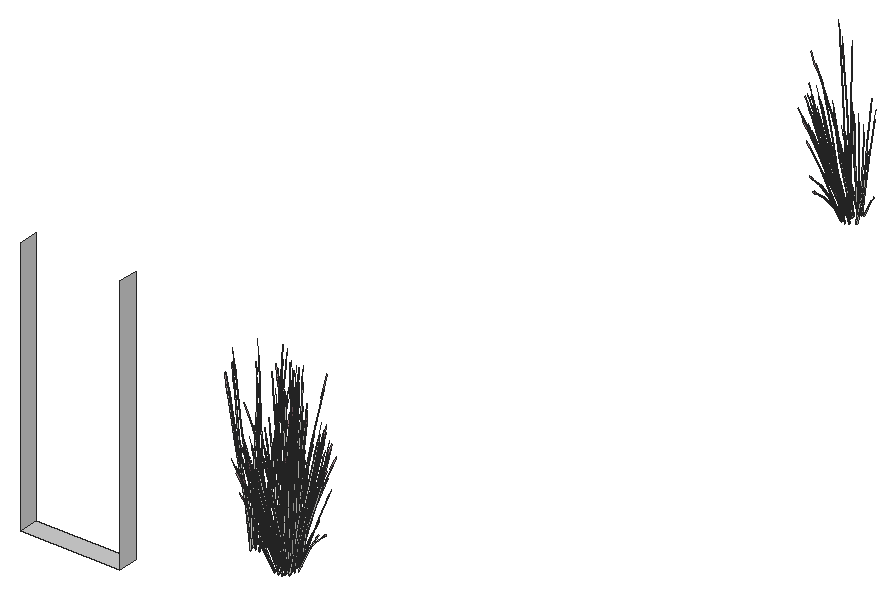
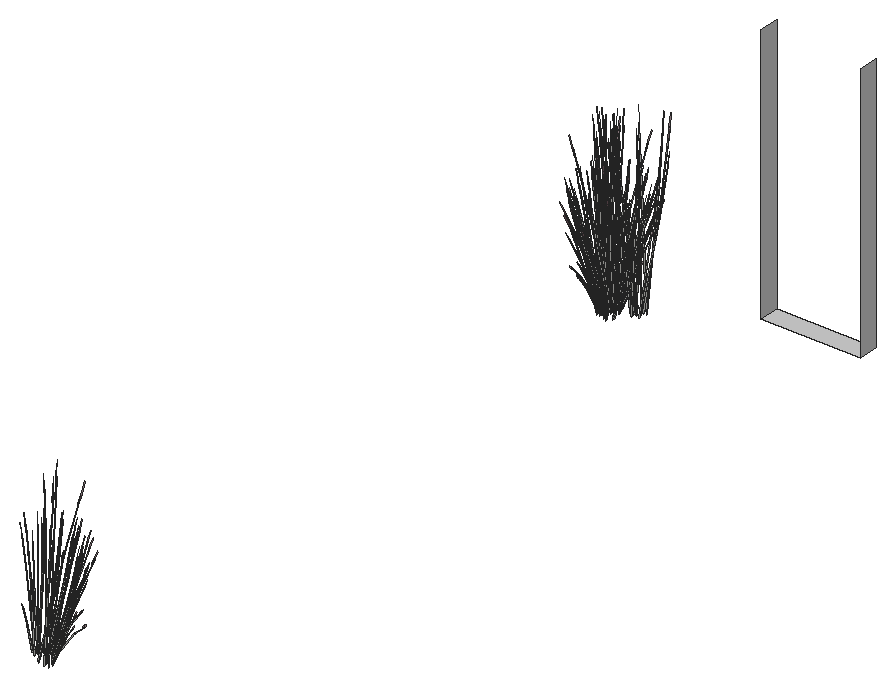
# SketchUp Ruby script. Lengths in inches.
U = 1.inch
M = Sketchup.active_model
def pt(a) = Geom::Point3d.new(a.map { |v| v * U })
def face(e, loops, mat)
  f = e.add_face(loops[0].map { |a| pt(a) })
  loops[1..].each { |l| e.add_face(l.map { |a| pt(a) }).erase! }
  f.material = f.back_material = mat if mat
  f
end
# faces: each face lists its corners as indices into pts; further lists are holes
def faces(e, pts, list, mat = nil) = list.each { |f| face(e, (f[0].is_a?(Array) ? f : [f]).map { |l| l.map { |i| pts[i] } }, mat) }
# xy, xz, yz: faces in a plane at the given z, y or x. An outline is a flat list of corners, or four numbers for a rectangle; further outlines are holes
def ring(l) = l.size == 4 ? [[l[0], l[1]], [l[2], l[1]], [l[2], l[3]], [l[0], l[3]]] : l.each_slice(2).to_a
def flat(e, list, mat, &to3) = list.each { |f| face(e, (f[0].is_a?(Array) ? f : [f]).map { |l| ring(l).map { |u, v| to3.(u, v) } }, mat) }
def xy(e, z, list, mat = nil) = flat(e, list, mat) { |x, y| [x, y, z] }
def xz(e, y, list, mat = nil) = flat(e, list, mat) { |x, z| [x, y, z] }
def yz(e, x, list, mat = nil) = flat(e, list, mat) { |y, z| [x, y, z] }
def lines(e, pts, list) = list.each { |a, b| e.add_line(pt(pts[a]), pt(pts[b])) }
# prism: a flat outline (further loops are holes) pulled along v
def prism(e, loops, v, mat = nil)
  f = face(e, loops, mat); d = Geom::Vector3d.new(v.map { |x| x * U })
  f.pushpull(f.normal.samedirection?(d) ? d.length : -d.length)
end
def box(e, o, s, mat = nil) = prism(e, [[o, [o[0] + s[0], o[1], o[2]], [o[0] + s[0], o[1] + s[1], o[2]], [o[0], o[1] + s[1], o[2]]]], [0, 0, s[2]], mat)
def at(x, y, z, deg = 0) = Geom::Transformation.translation(pt([x, y, z])) * Geom::Transformation.rotation(ORIGIN, Z_AXIS, deg.degrees)
def axes(o, x, y, z) = Geom::Transformation.new([*x, 0, *y, 0, *z, 0, *pt(o).to_a, 1])
def part(name) = M.definitions.add(name)
# library, detail: a bought-in or finely detailed component or shape, given as its bounding box
def library(name, o, s) = part(name).tap { |d| box(d.entities, o, s) }
def detail(e, o, s) = box(e.add_group.entities, o, s)
def put(e, d, t, mat = nil) = e.add_instance(d, t).tap { |i| i.material = mat if mat }
def group(e, t, mat = nil) = e.add_group.tap { |g| g.transformation = t; g.material = mat if mat }.entities
root = M.entities
M.materials.add("LightPink_Translucent").color = [144, 107, 117]
M.materials["LightPink_Translucent"].alpha = 0.75
M.materials.add("[Cladding_Siding_White]1").color = [207, 207, 207]
c1 = part("blade")
p = [[2.15,0.21,22],[0,0.17,0],[0.09,0.45,0],[2.18,0.31,22],[2.29,0.31,22],[0.38,0.45,0],
  [2.48,0.24,33],[2.49,0.24,33],[2.48,0.22,33]]
faces(c1.entities,p,[[0,1,2,3],[4,5,2,3],[6,3,4,7],[8,0,3,6]])
c2 = part("seeds")
p = [[0.3,-0.1,1.38],[-0.01,-0.03,1.59],[-0.01,-0.03,0.03],[0.14,-0.07,-0.07],[0.29,-0.03,3],[0.15,0.01,3.11]]
faces(c2.entities,p,[[0,1,2,3],[1,0,4,5]],"LightPink_Translucent")
c3 = part("blade with seeds")
put(c3.entities,c1,at(0,0,0))
put(c3.entities,c2,axes([2.4,0.25,30.99],[1.5799,-0.05474,1.17369],[-0.12525,1.92788,0.29478],[-0.07173,-0.02425,1.56792]))
xy(root,153,[[312,87,342,93]],"[Cladding_Siding_White]1")
yz(root,312,[[87,153,93,231]],"[Cladding_Siding_White]1")
yz(root,342,[[87,153,93,231]],"[Cladding_Siding_White]1")
put(root,c3,axes([371.09,110.03,153.64],[0.11194,0.19382,1.61094],[-0.51725,0.16318,0.13026],[-0.1169,-0.30428,0.68866]))
put(root,c3,axes([373.11,109.75,152.44],[-0.13919,0.12219,1.34422],[-0.41687,-0.21387,-0.28909],[0.07727,-0.26598,0.57472]))
put(root,c3,axes([372.47,110.17,154.68],[-0.23372,-0.49086,-0.66783],[0.48111,-0.27356,0.08059],[-0.05465,-0.23717,0.9447]))
put(root,c3,axes([370.95,109.51,152.44],[-0.02965,0.19748,1.34422],[-0.43351,0.16532,-0.28909],[-0.10133,-0.25525,0.57472]))
put(root,c3,axes([373.45,110.65,154.68],[0.01274,-0.55841,-0.66783],[0.53656,0.0375,0.08059],[0.05662,-0.23657,0.9447]))
put(root,c3,axes([372.52,109.75,154.25],[0.14763,-0.46424,-0.33289],[0.4307,0.1354,0.42977],[-0.03949,-0.18691,0.82232]))
put(root,c3,axes([372.84,110.37,153.64],[-0.09118,0.2075,1.61094],[-0.3825,-0.42941,0.13026],[0.17255,-0.26763,0.68866]))
put(root,c3,axes([372.3,110.07,154.4],[-0.48137,-0.15133,-0.48033],[0.165,-0.51886,-0.37205],[-0.04414,-0.2089,0.91906]))
put(root,c3,axes([372.59,108.77,152.6],[0.06282,0.35202,1.07969],[-0.34848,-0.19497,0.79328],[0.0375,-0.18025,0.23781]))
put(root,c3,axes([373.34,110.46,154.4],[-0.35055,-0.40562,-0.48033],[0.37031,-0.35523,-0.37205],[0.05334,-0.20609,0.91906]))
put(root,c3,axes([372.71,110.05,154.73],[-0.47919,0.28106,-0.11431],[-0.23549,-0.49884,-0.63445],[-0.06322,-0.21021,0.96403]))
put(root,c3,axes([373.7,110.68,154.73],[-0.53819,-0.02991,-0.11431],[0.01471,-0.56632,-0.63445],[0.03738,-0.21811,0.96403]))
put(root,c3,axes([373.67,110.31,154.25],[0.33133,-0.31784,-0.33289],[0.31365,0.36292,0.42977],[0.04772,-0.1844,0.82232]))
put(root,c3,axes([370.8,109.2,152.6],[0.25544,0.21011,1.07969],[-0.37201,0.1263,0.79328],[-0.0796,-0.16148,0.23781]))
put(root,c3,axes([371.42,110.31,154.68],[-0.41756,-0.29179,-0.66783],[0.29675,-0.51132,0.08059],[-0.15128,-0.17422,0.9447]))
put(root,c3,axes([371.28,109.92,154.25],[-0.07563,-0.48625,-0.33289],[0.43235,-0.1284,0.42977],[-0.11613,-0.13934,0.82232]))
put(root,c3,axes([362.35,112.01,155.67],[-0.2011,-0.61905,-0.65645],[0.5793,-0.22295,-0.17229],[-0.02223,-0.20963,1.449]))
put(root,c3,axes([370.34,110.63,153.64],[0.1819,0.10401,1.61094],[-0.37643,0.43634,0.13026],[-0.23461,-0.19684,0.68866]))
put(root,c3,axes([371.22,110.32,154.4],[-0.48321,0.1435,-0.48033],[-0.08453,-0.54345,-0.37205],[-0.12979,-0.15574,0.91906]))
put(root,c3,axes([374.08,111.62,154.68],[0.25579,-0.47633,-0.66783],[0.44823,0.33852,0.08059],[0.15273,-0.17258,0.9447]))
put(root,c3,axes([374.07,111.4,154.4],[-0.1258,-0.55122,-0.48033],[0.4764,-0.09643,-0.37205],[0.13652,-0.14806,0.91906]))
put(root,c3,axes([374.29,111.79,154.73],[-0.45297,-0.33287,-0.11431],[0.26096,-0.48206,-0.63445],[0.12798,-0.16757,0.96403]))
put(root,c3,axes([372.42,113.61,153.125],[0.42317,0.24343,1.42185],[-0.41456,0.52443,0.56227],[-0.18569,-0.31082,1.19198]))
put(root,c3,axes([361.17,111.93,155.59],[0,-0.60368,-0.46672],[0.54787,0,0],[0,-0.13749,1.48054]))
put(root,c3,axes([362.6875,110.14,155.59],[0.4583,-0.30184,-0.46672],[0.27394,0.54125,0],[0.10438,-0.06875,1.48054]))
put(root,c3,axes([374.45,111.18,152.44],[-0.17494,-0.01788,1.34422],[-0.17922,-0.47967,-0.28909],[0.21491,-0.13569,0.57472]))
put(root,c3,axes([363.23,111.38,155.63],[0.32983,-0.45375,-0.58612],[0.40974,0.41145,-0.15383],[0.13217,-0.11319,1.29375]))
put(root,c3,axes([374.65,110.3,152.6],[-0.16311,0.3073,1.07969],[-0.1402,-0.41288,0.79328],[0.13471,-0.10346,0.23781]))
put(root,c3,axes([374.42,111.46,154.25],[0.42626,-0.08628,-0.33289],[0.11256,0.4932,0.42977],[0.12215,-0.13247,0.82232]))
put(root,c3,axes([370.27,110.78,154.25],[-0.27863,-0.37797,-0.33289],[0.31815,-0.35779,0.42977],[-0.16164,-0.05444,0.82232]))
put(root,c3,axes([370.17,111.18,152.44],[0.09561,0.16807,1.34422],[-0.22031,0.45686,-0.28909],[-0.22622,-0.1092,0.57472]))
put(root,c3,axes([370.57,111.03,154.68],[-0.48951,-0.01454,-0.66783],[0.03288,-0.61207,0.08059],[-0.20738,-0.06459,0.9447]))
put(root,c3,axes([375.65,112.24,154.43],[0.06795,-0.09195,1.64448],[-0.08698,-0.56405,-0.26007],[0.1705,-0.10694,0.13189]))
put(root,c3,axes([370.41,111.15,154.4],[-0.35558,0.39989,-0.48033],[-0.31141,-0.42243,-0.37205],[-0.18066,-0.06084,0.91906]))
put(root,c3,axes([369.61,111.68,152.6],[0.31263,-0.0432,1.07969],[-0.19831,0.38061,0.79328],[-0.15449,-0.0571,0.23781]))
put(root,c3,axes([371.8125,112.04,152.56],[-0.53176,0.03727,0.42055],[-0.04809,-0.6186,-0.2024],[0.0952,-0.0627,1.35025]))
put(root,c3,axes([370.59,110.74,154.73],[-0.02622,0.61393,-0.11431],[-0.49645,-0.01678,-0.63445],[-0.1912,-0.04265,0.96403]))
put(root,c3,axes([370.44,112.49,152.33],[0,0.60368,0.46672],[-0.54787,0,0],[0,-0.13749,1.48054]))
put(root,c3,axes([374.31,113.09,154.73],[-0.24639,-0.54664,-0.11431],[0.43729,-0.26863,-0.63445],[0.18428,-0.07212,0.96403]))
put(root,c3,axes([374.29,112.62,154.4],[0.13266,-0.54912,-0.48033],[0.45484,0.18822,-0.37205],[0.18313,-0.05035,0.91906]))
put(root,c3,axes([369.96,111.58,153.64],[0.20312,-0.01367,1.61094],[-0.13474,0.59258,0.13026],[-0.28946,-0.03665,0.68866]))
put(root,c3,axes([371.6875,112.79,152.56],[-0.23759,0.54397,0.42055],[-0.49367,-0.26179,-0.2024],[0,-0.12539,1.35025]))
put(root,c3,axes([373.3,110.7,152.33],[-0.4583,-0.30184,0.46672],[0.27394,-0.54125,0],[0.10438,0.06875,1.48054]))
put(root,c3,axes([374.2,112.82,154.68],[0.4303,-0.26662,-0.66783],[0.23981,0.54882,0.08059],[0.20791,-0.06234,0.9447]))
put(root,c3,axes([362.43,113.17,155.63],[-0.50939,-0.09897,-0.58612],[0.10749,-0.61051,-0.15383],[-0.15202,-0.07398,1.29375]))
put(root,c3,axes([371.57,110.97,152.33],[-0.14146,0.59996,0.16584],[-0.51766,-0.16978,0.32981],[0.08942,-0.00292,1.50782]))
put(root,c3,axes([372.65,111.64,152.46],[0.09447,-0.53876,0.13611],[0.46155,0.09352,-0.38866],[0.084,0.05532,1.1914]))
put(root,c3,axes([372.45,111.78,152.56],[-0.29417,-0.5067,0.42055],[0.44558,-0.35681,-0.2024],[0.0952,0.0627,1.35025]))
put(root,c3,axes([371.52,114.07,152.33],[0.52621,-0.16023,0.16584],[0.12993,0.59629,0.32981],[-0.04693,-0.08688,1.50782]))
put(root,c3,axes([374.57,112.875,154.25],[0.40696,0.16841,-0.33289],[-0.1187,0.49132,0.42977],[0.16385,-0.04505,0.82232]))
put(root,c3,axes([361.76,114.32,155.59],[-0.4583,-0.30184,-0.46672],[0.27394,-0.54125,0],[-0.10438,-0.06875,1.48054]))
put(root,c3,axes([364.81,110.75,155.59],[0.4583,0.30184,-0.46672],[-0.27394,0.54125,0],[0.10438,0.06875,1.48054]))
put(root,c3,axes([369.78,112.09,154.25],[-0.40696,-0.16841,-0.33289],[0.1187,-0.49132,0.42977],[-0.16385,0.04505,0.82232]))
put(root,c3,axes([373.13,111.01,152.33],[-0.52621,0.16023,0.16584],[-0.12993,-0.59629,0.32981],[0.04693,0.08688,1.50782]))
put(root,c3,axes([373.46,112.26,153.64],[-0.20312,0.01367,1.61094],[0.13474,-0.59258,0.13026],[0.28946,0.03665,0.68866]))
put(root,c3,axes([372,113.43,152.46],[-0.09447,0.53876,0.13611],[-0.46155,-0.09352,-0.38866],[-0.084,-0.05532,1.1914]))
put(root,c3,axes([373.08,114.1,152.33],[0.14146,-0.59996,0.16584],[0.51766,0.16978,0.32981],[-0.08942,0.00292,1.50782]))
put(root,c3,axes([371.02,112.01,153.14],[0.13919,-0.08733,1.6644],[0.048,0.60974,0.13026],[-0.3015,0.08091,0.59487]))
put(root,c3,axes([373.89,112.57,152.33],[-0.38474,-0.43973,0.16584],[0.38772,-0.42651,0.32981],[-0.04249,0.0898,1.50782]))
put(root,c3,axes([364.14,111.91,155.63],[0.50939,0.09897,-0.58612],[-0.10749,0.61051,-0.15383],[0.15202,0.07398,1.29375]))
put(root,c3,axes([375.43,112.97,152.6],[-0.30256,0.09966,1.07969],[0.14242,-0.41189,0.79328],[0.16051,0.02818,0.23781]))
put(root,c3,axes([371.35,114.375,152.33],[0.4583,0.30184,0.46672],[-0.27394,0.54125,0],[-0.10438,-0.06875,1.48054]))
put(root,c3,axes([372.96,112.28,152.56],[0.23759,-0.54397,0.42055],[0.49367,0.26179,-0.2024],[0,0.12539,1.35025]))
put(root,c3,axes([369.53,112.42,154.43],[-0.07997,0.07838,1.64448],[0.0068,0.57266,-0.26007],[-0.1833,0.07447,0.13189]))
put(root,c3,axes([370.0625,112.34,154.4],[-0.13266,0.54912,-0.48033],[-0.45484,-0.18822,-0.37205],[-0.18313,0.05035,0.91906]))
put(root,c3,axes([370.04,111.87,154.73],[0.24639,0.54664,-0.11431],[-0.43729,0.26863,-0.63445],[-0.18428,0.07212,0.96403]))
put(root,c3,axes([374.9,114.24,153.69],[-0.09372,-0.50747,-0.03282],[0.44299,-0.11666,-0.14882],[0.09251,0.03217,0.49085]))
put(root,c3,axes([373.75,114.23,154.73],[0.02622,-0.61393,-0.11431],[0.49645,0.01678,-0.63445],[0.1912,0.04265,0.96403]))
put(root,c3,axes([374.21,112.59,152.33],[0,-0.60368,0.46672],[0.54787,0,0],[0,0.13749,1.48054]))
put(root,c3,axes([372.83,113.04,152.56],[0.53176,-0.03727,0.42055],[0.04809,0.6186,-0.2024],[-0.0952,0.0627,1.35025]))
put(root,c3,axes([373.17,112.41,152.46],[0.45625,-0.17605,0.13611],[0.15978,0.50273,-0.38866],[0,0.11064,1.1914]))
put(root,c3,axes([374.86,113.63,152.44],[-0.11793,-0.14847,1.34422],[0.15345,-0.49116,-0.28909],[0.23861,0.06653,0.57472]))
put(root,c3,axes([374.1875,113.86,154.43],[0.10505,-0.01021,1.64448],[0.28813,-0.469,-0.26007],[0.18685,0.06191,0.13189]))
put(root,c3,axes([372.84,113.31,152.46],[0.36178,0.36271,0.13611],[-0.30177,0.40921,-0.38866],[-0.084,0.05532,1.1914]))
put(root,c3,axes([370.05,112.625,153.64],[0.16991,-0.12769,1.61094],[0.14304,0.59005,0.13026],[-0.26674,0.13336,0.68866]))
put(root,c3,axes([373.78,113.93,154.68],[0.48951,0.01454,-0.66783],[-0.03288,0.61207,0.08059],[0.20738,0.06459,0.9447]))
put(root,c3,axes([373.23,114.42,152.33],[0.4583,-0.30184,0.46672],[0.27394,0.54125,0],[-0.10438,0.06875,1.48054]))
put(root,c3,axes([369.52,113.63,152.44],[0.17018,0.04956,1.34422],[0.10969,0.50618,-0.28909],[-0.23117,0.09475,0.57472]))
put(root,c3,axes([369.16,114.69,152.6],[0.20408,-0.2736,1.07969],[0.08053,0.43313,0.79328],[-0.14748,0.07756,0.23781]))
put(root,c3,axes([374.07,114.18,154.25],[0.27863,0.37797,-0.33289],[-0.31815,0.35779,0.42977],[0.16164,0.05444,0.82232]))
put(root,c3,axes([369.93,113.51,154.25],[-0.42626,0.08628,-0.33289],[-0.11256,-0.4932,0.42977],[-0.12215,0.13247,0.82232]))
put(root,c3,axes([363.34,113.7,155.63],[-0.32983,0.45375,-0.58612],[-0.40974,-0.41145,-0.15383],[-0.13217,0.11319,1.29375]))
put(root,c3,axes([363.88,114.94,155.59],[-0.4583,0.30184,-0.46672],[-0.27394,-0.54125,0],[-0.10438,0.06875,1.48054]))
put(root,c3,axes([365.4,113.15,155.59],[0,0.60368,-0.46672],[-0.54787,0,0],[0,0.13749,1.48054]))
put(root,c3,axes([373.07,113.22,153.64],[-0.1819,-0.10401,1.61094],[0.37643,-0.43634,0.13026],[0.23461,0.19684,0.68866]))
put(root,c3,axes([373.11,111.85,154.21],[-0.42314,-0.31366,1.29986],[0.4468,-0.48836,0.56085],[0.13652,0.29431,1.25644]))
put(root,c3,axes([370.06,113.17,154.73],[0.45297,0.33287,-0.11431],[-0.26096,0.48206,-0.63445],[-0.12798,0.16757,0.96403]))
put(root,c3,axes([373.75,114.4,152.6],[-0.27572,-0.17358,1.07969],[0.35602,-0.17637,0.79328],[0.09603,0.1494,0.23781]))
put(root,c3,axes([372.78,114.9,154.73],[0.2918,-0.51673,-0.11431],[0.42258,0.29769,-0.63445],[0.14689,0.14599,0.96403]))
put(root,c3,axes([370.67,113.02,153.64],[0.12231,-0.18549,1.61094],[0.30882,0.50067,0.13026],[-0.21182,0.22801,0.68866]))
put(root,c3,axes([370.28,113.56,154.4],[0.1258,0.55122,-0.48033],[-0.4764,0.09643,-0.37205],[-0.13652,0.14806,0.91906]))
put(root,c3,axes([373.07,112.45,152.67],[-0.01338,-0.56839,1.32796],[0.60542,0.14734,0.56227],[-0.14319,0.31102,1.25349]))
put(root,c3,axes([364.19,113.07,155.67],[0.17956,0.55272,-0.65059],[-0.51723,0.19906,-0.17075],[0.01985,0.18717,1.43607]))
put(root,c3,axes([373.125,114.64,154.4],[0.48321,-0.1435,-0.48033],[0.08453,0.54345,-0.37205],[0.12979,0.15574,0.91906]))
put(root,c3,axes([373.79,115.19,152.51],[-0.31402,-0.01893,0.98757],[0.20738,-0.40212,0.54525],[0.12405,0.14286,0.77466]))
put(root,c3,axes([370.58,113.48,153.64],[0.09118,-0.2075,1.61094],[0.3825,0.42941,0.13026],[-0.17255,0.26763,0.68866]))
put(root,c3,axes([372.77,114.22,152.44],[0.00864,-0.20012,1.34422],[0.41296,-0.22353,-0.28909],[0.12748,0.23952,0.57472]))
put(root,c3,axes([370.68,114.65,154.25],[-0.33133,0.31784,-0.33289],[-0.31365,-0.36292,0.42977],[-0.04772,0.1844,0.82232]))
put(root,c3,axes([371.64,114.92,154.73],[0.47919,-0.28106,-0.11431],[0.23549,0.49884,-0.63445],[0.06322,0.21021,0.96403]))
put(root,c3,axes([370.89,115.88,152.6],[-0.01267,-0.35895,1.07969],[0.31667,0.25602,0.79328],[-0.06228,0.17109,0.23781]))
put(root,c3,axes([371.01,114.5,154.7],[0.35055,0.40562,-0.53317],[-0.37031,0.35523,-0.41298],[-0.05334,0.20609,1.02016]))
put(root,c3,axes([370.63,115.11,152.65],[0.44486,-0.1069,0.06117],[0.10227,0.43069,-0.81126],[-0.0282,0.21802,0.72719]))
put(root,c3,axes([372.05,114.89,154.4],[0.48137,0.15133,-0.48033],[-0.165,0.51886,-0.37205],[0.04414,0.2089,0.91906]))
put(root,c3,axes([372.32,113.82,153.64],[-0.11194,-0.19382,1.61094],[0.51725,-0.16318,0.13026],[0.1169,0.30428,0.68866]))
put(root,c3,axes([371.83,115.21,154.25],[-0.14763,0.46424,-0.33289],[-0.4307,-0.1354,0.42977],[0.03949,0.18691,0.82232]))
put(root,c3,axes([370.9,114.3125,155.02],[-0.01274,0.55841,-0.74129],[-0.53656,-0.0375,0.08946],[-0.05662,0.23657,1.04862]))
put(root,c3,axes([371.41,113.92,153.64],[-0.01199,-0.2317,1.61094],[0.51947,0.15371,0.13026],[-0.03213,0.3302,0.68866]))
put(root,c3,axes([371.875,114.79,154.68],[0.23372,0.49086,-0.66783],[-0.48111,0.27356,0.08059],[0.05465,0.23717,0.9447]))
put(root,c3,axes([370.52,115.57,152.44],[0.15453,-0.09523,1.34422],[0.38153,0.28715,-0.28909],[-0.11356,0.24846,0.57472]))
put(root,c3,axes([370.72,115.1,153.16],[0.01076,-0.31164,1.45085],[0.48391,0.16461,0.20049],[-0.04193,0.33214,0.68509]))
put(root,c3,axes([369.83,325.32,153.64],[0.11194,0.19382,1.61094],[-0.51725,0.16318,0.13026],[-0.1169,-0.30428,0.68866]))
put(root,c3,axes([370.6875,324.03,154.43],[-0.0749,-0.08464,1.64448],[-0.49984,0.05366,-0.26007],[-0.07977,-0.20245,0.13189]))
put(root,c3,axes([371.85,325.04,152.44],[-0.13919,0.12219,1.34422],[-0.41687,-0.21387,-0.28909],[0.07727,-0.26598,0.57472]))
put(root,c3,axes([371.21,325.46,154.68],[-0.23372,-0.49086,-0.66783],[0.48111,-0.27356,0.08059],[-0.05465,-0.23717,0.9447]))
put(root,c3,axes([369.69,324.81,152.44],[-0.02965,0.19748,1.34422],[-0.43351,0.16532,-0.28909],[-0.10133,-0.25525,0.57472]))
put(root,c3,axes([372.1875,325.94,154.68],[0.01274,-0.55841,-0.66783],[0.53656,0.0375,0.08059],[0.05662,-0.23657,0.9447]))
put(root,c3,axes([372.93,325.07,154.43],[-0.00473,-0.12015,1.64448],[-0.39924,-0.34724,-0.26007],[0.06173,-0.21049,0.13189]))
put(root,c3,axes([371.26,325.04,154.25],[0.14763,-0.46424,-0.33289],[0.4307,0.1354,0.42977],[-0.03949,-0.18691,0.82232]))
put(root,c3,axes([371.58,325.66,153.64],[-0.09118,0.2075,1.61094],[-0.3825,-0.42941,0.13026],[0.17255,-0.26763,0.68866]))
put(root,c3,axes([371.04,325.36,154.4],[-0.48137,-0.15133,-0.48033],[0.165,-0.51886,-0.37205],[-0.04414,-0.2089,0.91906]))
put(root,c3,axes([371.33,324.0625,152.6],[0.06282,0.35202,1.07969],[-0.34848,-0.19497,0.79328],[0.0375,-0.18025,0.23781]))
put(root,c3,axes([372.08,325.76,154.4],[-0.35055,-0.40562,-0.48033],[0.37031,-0.35523,-0.37205],[0.05334,-0.20609,0.91906]))
put(root,c3,axes([371.45,325.34,154.73],[-0.47919,0.28106,-0.11431],[-0.23549,-0.49884,-0.63445],[-0.06322,-0.21021,0.96403]))
put(root,c3,axes([372.44,325.97,154.73],[-0.53819,-0.02991,-0.11431],[0.01471,-0.56632,-0.63445],[0.03738,-0.21811,0.96403]))
put(root,c3,axes([372.41,325.61,154.25],[0.33133,-0.31784,-0.33289],[0.31365,0.36292,0.42977],[0.04772,-0.1844,0.82232]))
put(root,c3,axes([369.54,324.49,152.6],[0.25544,0.21011,1.07969],[-0.37201,0.1263,0.79328],[-0.0796,-0.16148,0.23781]))
put(root,c3,axes([370.16,325.6,154.68],[-0.41756,-0.29179,-0.66783],[0.29675,-0.51132,0.08059],[-0.15128,-0.17422,0.9447]))
put(root,c3,axes([370.02,325.21,154.25],[-0.07563,-0.48625,-0.33289],[0.43235,-0.1284,0.42977],[-0.11613,-0.13934,0.82232]))
put(root,c3,axes([369.08,325.92,153.64],[0.1819,0.10401,1.61094],[-0.37643,0.43634,0.13026],[-0.23461,-0.19684,0.68866]))
put(root,c3,axes([369.96,325.62,154.4],[-0.48321,0.1435,-0.48033],[-0.08453,-0.54345,-0.37205],[-0.12979,-0.15574,0.91906]))
put(root,c3,axes([372.82,326.91,154.68],[0.25579,-0.47633,-0.66783],[0.44823,0.33852,0.08059],[0.15273,-0.17258,0.9447]))
put(root,c3,axes([372.81,326.69,154.4],[-0.1258,-0.55122,-0.48033],[0.4764,-0.09643,-0.37205],[0.13652,-0.14806,0.91906]))
put(root,c3,axes([369.05,324.96,154.43],[-0.10536,-0.00426,1.64448],[-0.33544,0.42612,-0.26007],[-0.17898,-0.08707,0.13189]))
put(root,c3,axes([373.03,327.08,154.73],[-0.45297,-0.33287,-0.11431],[0.26096,-0.48206,-0.63445],[0.12798,-0.16757,0.96403]))
put(root,c3,axes([371.16,328.9,153.125],[0.42317,0.24343,1.42185],[-0.41456,0.52443,0.56227],[-0.18569,-0.31082,1.19198]))
put(root,c3,axes([373.1875,326.47,152.44],[-0.17494,-0.01788,1.34422],[-0.17922,-0.47967,-0.28909],[0.21491,-0.13569,0.57472]))
put(root,c3,axes([373.39,325.59,152.6],[-0.16311,0.3073,1.07969],[-0.1402,-0.41288,0.79328],[0.13471,-0.10346,0.23781]))
put(root,c3,axes([373.16,326.75,154.25],[0.42626,-0.08628,-0.33289],[0.11256,0.4932,0.42977],[0.12215,-0.13247,0.82232]))
put(root,c3,axes([369.01,326.07,154.25],[-0.27863,-0.37797,-0.33289],[0.31815,-0.35779,0.42977],[-0.16164,-0.05444,0.82232]))
put(root,c3,axes([368.91,326.47,152.44],[0.09561,0.16807,1.34422],[-0.22031,0.45686,-0.28909],[-0.22622,-0.1092,0.57472]))
put(root,c3,axes([369.31,326.32,154.68],[-0.48951,-0.01454,-0.66783],[0.03288,-0.61207,0.08059],[-0.20738,-0.06459,0.9447]))
put(root,c3,axes([374.39,327.53,154.43],[0.06795,-0.09195,1.64448],[-0.08698,-0.56405,-0.26007],[0.1705,-0.10694,0.13189]))
put(root,c3,axes([369.15,326.45,154.4],[-0.35558,0.39989,-0.48033],[-0.31141,-0.42243,-0.37205],[-0.18066,-0.06084,0.91906]))
put(root,c3,axes([368.34,326.98,152.6],[0.31263,-0.0432,1.07969],[-0.19831,0.38061,0.79328],[-0.15449,-0.0571,0.23781]))
put(root,c3,axes([370.55,327.33,152.56],[-0.53176,0.03727,0.42055],[-0.04809,-0.6186,-0.2024],[0.0952,-0.0627,1.35025]))
put(root,c3,axes([369.33,326.03,154.73],[-0.02622,0.61393,-0.11431],[-0.49645,-0.01678,-0.63445],[-0.1912,-0.04265,0.96403]))
put(root,c3,axes([369.18,327.78,152.33],[0,0.60368,0.46672],[-0.54787,0,0],[0,-0.13749,1.48054]))
put(root,c3,axes([373.05,328.38,154.73],[-0.24639,-0.54664,-0.11431],[0.43729,-0.26863,-0.63445],[0.18428,-0.07212,0.96403]))
put(root,c3,axes([373.03,327.91,154.4],[0.13266,-0.54912,-0.48033],[0.45484,0.18822,-0.37205],[0.18313,-0.05035,0.91906]))
put(root,c3,axes([368.7,326.87,153.64],[0.20312,-0.01367,1.61094],[-0.13474,0.59258,0.13026],[-0.28946,-0.03665,0.68866]))
put(root,c3,axes([370.43,328.08,152.56],[-0.23759,0.54397,0.42055],[-0.49367,-0.26179,-0.2024],[0,-0.12539,1.35025]))
